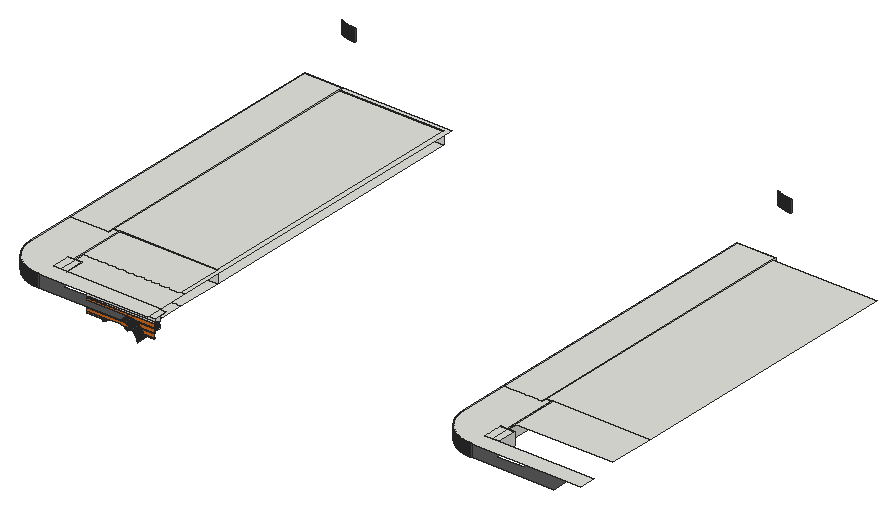
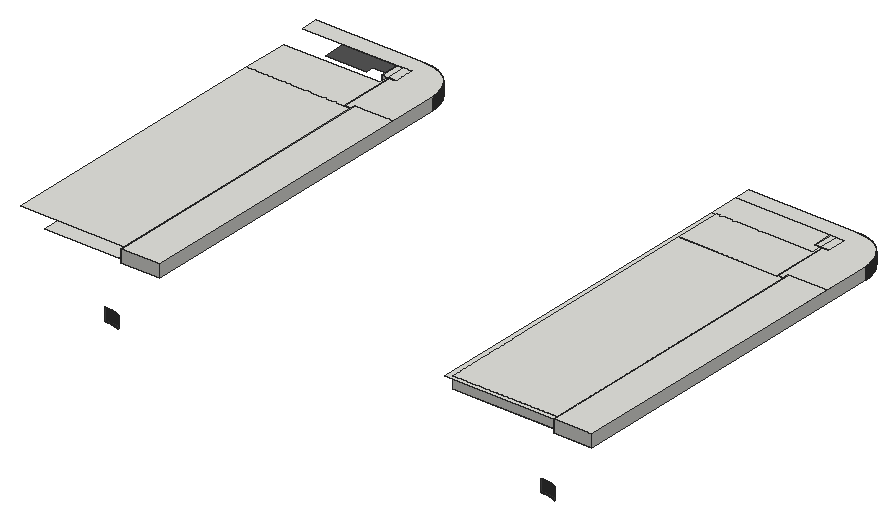
# SketchUp Ruby script. Lengths in inches.
U = 1.inch
M = Sketchup.active_model
def pt(a) = Geom::Point3d.new(a.map { |v| v * U })
def face(e, loops, mat)
  f = e.add_face(loops[0].map { |a| pt(a) })
  loops[1..].each { |l| e.add_face(l.map { |a| pt(a) }).erase! }
  f.material = f.back_material = mat if mat
  f
end
# faces: each face lists its corners as indices into pts; further lists are holes
def faces(e, pts, list, mat = nil) = list.each { |f| face(e, (f[0].is_a?(Array) ? f : [f]).map { |l| l.map { |i| pts[i] } }, mat) }
# xy, xz, yz: faces in a plane at the given z, y or x. An outline is a flat list of corners, or four numbers for a rectangle; further outlines are holes
def ring(l) = l.size == 4 ? [[l[0], l[1]], [l[2], l[1]], [l[2], l[3]], [l[0], l[3]]] : l.each_slice(2).to_a
def flat(e, list, mat, &to3) = list.each { |f| face(e, (f[0].is_a?(Array) ? f : [f]).map { |l| ring(l).map { |u, v| to3.(u, v) } }, mat) }
def xy(e, z, list, mat = nil) = flat(e, list, mat) { |x, y| [x, y, z] }
def xz(e, y, list, mat = nil) = flat(e, list, mat) { |x, z| [x, y, z] }
def yz(e, x, list, mat = nil) = flat(e, list, mat) { |y, z| [x, y, z] }
def lines(e, pts, list) = list.each { |a, b| e.add_line(pt(pts[a]), pt(pts[b])) }
# prism: a flat outline (further loops are holes) pulled along v
def prism(e, loops, v, mat = nil)
  f = face(e, loops, mat); d = Geom::Vector3d.new(v.map { |x| x * U })
  f.pushpull(f.normal.samedirection?(d) ? d.length : -d.length)
end
def box(e, o, s, mat = nil) = prism(e, [[o, [o[0] + s[0], o[1], o[2]], [o[0] + s[0], o[1] + s[1], o[2]], [o[0], o[1] + s[1], o[2]]]], [0, 0, s[2]], mat)
def at(x, y, z, deg = 0) = Geom::Transformation.translation(pt([x, y, z])) * Geom::Transformation.rotation(ORIGIN, Z_AXIS, deg.degrees)
def axes(o, x, y, z) = Geom::Transformation.new([*x, 0, *y, 0, *z, 0, *pt(o).to_a, 1])
def part(name) = M.definitions.add(name)
# library, detail: a bought-in or finely detailed component or shape, given as its bounding box
def library(name, o, s) = part(name).tap { |d| box(d.entities, o, s) }
def detail(e, o, s) = box(e.add_group.entities, o, s)
def put(e, d, t, mat = nil) = e.add_instance(d, t).tap { |i| i.material = mat if mat }
def group(e, t, mat = nil) = e.add_group.tap { |g| g.transformation = t; g.material = mat if mat }.entities
root = M.entities
M.materials.add("[0041_Chocolate]").color = [210, 105, 30]
M.materials.add("[Color M06]").color = [84, 84, 84]
xy(root,385.02,[[897.21,280.47,926.7,281.47],[954.52,280.47,998.64,281.47]],"[0041_Chocolate]")
xy(root,386.9375,[[897.21,280.47,931.67,281.47],[949.56,280.47,998.64,281.47]],"[0041_Chocolate]")
xy(root,391.89,[[897.21,280.47,998.64,281.47]],"[0041_Chocolate]")
xy(root,393.8125,[[897.21,280.47,998.64,281.47]],"[0041_Chocolate]")
xy(root,395.26,[[897.21,302.46,976.46,310.27]])
xy(root,398.77,[[897.21,280.47,998.64,281.47]],"[0041_Chocolate]")
xy(root,400.6875,[[897.21,280.47,998.64,281.47]],"[0041_Chocolate]")
xy(root,402.64,[[897.21,300.33,958.42,302.46],[990.02,302.46,992.73,302.46,992.73,337.5625,845.71,337.5625,845.71,321.34,857.24,321.34,857.24,305.58,897.21,305.58,897.21,312.8125,990.02,312.8125],[897.21,302.46,990.02,312.8125],[836,305.58,845.71,312.8125],[845.71,305.58,857.24,312.8125],
  [1486.5,305.58,1496.21,312.8125],[1496.21,305.58,1507.74,312.8125],[836,312.8125,845.71,321.34],[845.71,312.8125,857.24,321.34],[1486.5,312.8125,1496.21,321.34],
  [1496.21,312.8125,1507.74,321.34],[845.71,337.5625,992.73,406.38],[844.53,399.07,845.71,406.38],[1495.03,399.07,1496.21,406.38],[836,406.38,844.53,830.91],
  [844.53,406.38,955.73,830.91],[955.73,406.38,992.73,830.91],[1486.5,406.38,1495.03,830.91],[1495.03,406.38,1606.23,830.91]])
xy(root,402.64,[[834.95,267.75,833.46,267.77,831.97,267.83,830.49,267.93,829.01,268.0625,827.53,268.24,826.05,268.45,824.59,268.7,823.125,268.99,821.67,269.32,820.23,269.6875,818.8,270.09,817.375,270.53,815.96,271.01,814.57,271.53,813.18,272.08,811.8125,272.67,810.46,273.29,809.125,273.95,807.81,274.64,806.51,275.37,805.23,276.13,803.97,276.93,802.73,277.75,801.51,278.61,800.32,279.51,799.15,280.43,798.01,281.38,796.89,282.36,795.79,283.37,794.73,284.41,793.6875,285.48,792.68,286.57,791.69,287.69,790.74,288.84,789.82,290.01,788.93,291.2,788.07,292.42,787.24,293.65,786.45,294.91,785.6875,296.19,784.96,297.49,784.27,298.8125,783.61,300.15,782.98,301.5,782.4,302.87,781.84,304.25,781.33,305.65,780.85,307.06,780.41,308.48,780,309.91,779.64,311.36,779.31,312.81,779.02,314.27,778.77,315.74,778.55,317.21,778.375,318.69,778.24,320.17,778.14,321.66,778.08,323.15,778.07,324.64,778.07,838.14,836,838.14,836,305.58,857.24,305.58,857.24,287.95,897.21,287.95,897.21,300.33,958.42,300.33,958.42,267.75],[1485.45,267.75,1483.96,267.77,1482.47,267.83,1480.99,267.93,1479.51,268.0625,1478.03,268.24,1476.55,268.45,1475.09,268.7,1473.625,268.99,1472.17,269.32,1470.73,269.6875,1469.3,270.09,1467.875,270.53,1466.46,271.01,1465.07,271.53,1463.68,272.08,1462.3125,272.67,1460.96,273.29,1459.625,273.95,1458.31,274.64,1457.01,275.37,1455.73,276.13,1454.47,276.93,1453.23,277.75,1452.01,278.61,1450.82,279.51,1449.65,280.43,1448.51,281.38,1447.39,282.36,1446.29,283.37,1445.23,284.41,1444.1875,285.48,1443.18,286.57,1442.19,287.69,1441.24,288.84,1440.32,290.01,1439.43,291.2,1438.57,292.42,1437.74,293.65,1436.95,294.91,1436.1875,296.19,1435.46,297.49,1434.77,298.8125,1434.11,300.15,1433.48,301.5,1432.9,302.87,1432.34,304.25,1431.83,305.65,1431.35,307.06,1430.91,308.48,1430.5,309.91,1430.14,311.36,1429.81,312.81,1429.52,314.27,1429.27,315.74,1429.05,317.21,1428.875,318.69,1428.74,320.17,1428.64,321.66,1428.58,323.15,1428.57,324.64,1428.57,838.14,1486.5,838.14,1486.5,305.58,1507.74,305.58,1507.74,287.95,1547.71,287.95,1547.71,300.33,1608.92,300.33,1608.92,267.75]],"[Color M06]")
xy(root,405.64,[[897.21,280.47,998.64,281.47]],"[0041_Chocolate]")
xy(root,411.82,[[897.21,281.47,998.64,302.46]])
xy(root,421.25,[[834.95,267.75,999.52,267.75,999.52,292.45,836,292.45,836,321.34,844.53,321.34,844.53,406.38,836,406.38,836,397.86,778.07,397.86,778.07,324.64,778.08,323.15,778.14,321.66,778.24,320.17,778.375,318.69,778.55,317.21,778.77,315.74,779.02,314.27,779.31,312.81,779.64,311.36,780,309.91,780.41,308.48,780.85,307.06,781.33,305.65,781.84,304.25,782.4,302.87,782.98,301.5,783.61,300.15,784.27,298.8125,784.96,297.49,785.6875,296.19,786.45,294.91,787.24,293.65,788.07,292.42,788.93,291.2,789.82,290.01,790.74,288.84,791.69,287.69,792.68,286.57,793.6875,285.48,794.73,284.41,795.79,283.37,796.89,282.36,798.01,281.38,799.15,280.43,800.32,279.51,801.51,278.61,802.73,277.75,803.97,276.93,805.23,276.13,806.51,275.37,807.81,274.64,809.125,273.95,810.46,273.29,811.8125,272.67,813.18,272.08,814.57,271.53,815.96,271.01,817.375,270.53,818.8,270.09,820.23,269.6875,821.67,269.32,823.125,268.99,824.59,268.7,826.05,268.45,827.53,268.24,829.01,268.0625,830.49,267.93,831.97,267.83,833.46,267.77],[1485.45,267.75,1650.02,267.75,1650.02,292.45,1486.5,292.45,1486.5,321.34,1495.03,321.34,1495.03,406.38,1486.5,406.38,1486.5,397.86,1428.57,397.86,1428.57,324.64,1428.58,323.15,1428.64,321.66,1428.74,320.17,1428.875,318.69,1429.05,317.21,1429.27,315.74,1429.52,314.27,1429.81,312.81,1430.14,311.36,1430.5,309.91,1430.91,308.48,1431.35,307.06,1431.83,305.65,1432.34,304.25,1432.9,302.87,1433.48,301.5,1434.11,300.15,1434.77,298.8125,1435.46,297.49,1436.1875,296.19,1436.95,294.91,1437.74,293.65,1438.57,292.42,1439.43,291.2,1440.32,290.01,1441.24,288.84,1442.19,287.69,1443.18,286.57,1444.1875,285.48,1445.23,284.41,1446.29,283.37,1447.39,282.36,1448.51,281.38,1449.65,280.43,1450.82,279.51,1452.01,278.61,1453.23,277.75,1454.47,276.93,1455.73,276.13,1457.01,275.37,1458.31,274.64,1459.625,273.95,1460.96,273.29,1462.3125,272.67,1463.68,272.08,1465.07,271.53,1466.46,271.01,1467.875,270.53,1469.3,270.09,1470.73,269.6875,1472.17,269.32,1473.625,268.99,1475.09,268.7,1476.55,268.45,1478.03,268.24,1479.51,268.0625,1480.99,267.93,1482.47,267.83,1483.96,267.77],[836,292.45,847.59,321.34],[847.59,292.45,857.24,321.34],[857.24,292.45,999.52,292.45,999.52,336.27,847.59,336.27,847.59,321.34,857.24,321.34],
  [1486.5,292.45,1498.09,321.34],[1498.09,292.45,1507.74,321.34],[844.53,321.34,845.71,406.38],[845.71,321.34,847.59,321.34,847.59,336.27,992.73,336.27,992.73,406.38,845.71,406.38],[1495.03,321.34,1496.21,406.38],
  [1496.21,321.34,1498.09,321.34,1498.09,336.27,1643.23,336.27,1643.23,406.38,1496.21,406.38],[992.73,336.27,999.52,336.27,999.52,838.14,836,838.14,836,830.91,992.73,830.91],[778.07,397.86,836,838.14],[1428.57,397.86,1486.5,838.14],[836,406.38,992.73,830.91],
  [1486.5,406.38,1643.23,830.91]])
xz(root,280.47,[[897.21,386.9375,931.67,386.9375,936.5,388.23,944.69,388.24,949.56,386.9375,998.64,386.9375,998.64,391.89,897.21,391.89],[897.21,393.8125,998.64,398.77],[897.21,400.6875,998.64,405.64]],"[0041_Chocolate]")
xz(root,281.47,[[897.21,405.64,998.64,407.5625],[897.21,407.5625,998.64,411.82],[897.21,411.82,998.64,412.52]])
xz(root,281.47,[[897.21,385.02,926.7,385.02,928.6,386.11,931.67,386.9375,897.21,386.9375],[954.52,385.02,998.64,385.02,998.64,386.9375,949.56,386.9375,952.6,386.125],[897.21,391.89,998.64,393.8125],[897.21,398.77,998.64,400.6875]],"[0041_Chocolate]")
xz(root,302.46,[[897.21,395.26,976.46,395.26,976.15,395.5625,975.66,396.02,975.15,396.46,974.63,396.89,974.1,397.3125,973.56,397.72,973.01,398.1,972.45,398.48,971.88,398.84,971.3,399.18,970.71,399.51,970.11,399.83,969.51,400.125,968.9,400.41,968.28,400.67,967.65,400.92,967.02,401.16,966.38,401.375,965.74,401.57,965.09,401.76,964.43,401.92,963.77,402.07,963.11,402.2,962.45,402.32,961.78,402.41,961.11,402.49,960.44,402.56,959.77,402.6,959.09,402.625,958.42,402.64,897.21,402.64],[976.46,395.26,984.18,395.26,984.18,402.64,958.42,402.64,959.09,402.625,959.77,402.6,960.44,402.56,961.11,402.49,961.78,402.41,962.45,402.32,963.11,402.2,963.77,402.07,964.43,401.92,965.09,401.76,965.74,401.57,966.38,401.375,967.02,401.16,967.65,400.92,968.28,400.67,968.9,400.41,969.51,400.125,970.11,399.83,970.71,399.51,971.3,399.18,971.88,398.84,972.45,398.48,973.01,398.1,973.56,397.72,974.1,397.3125,974.63,396.89,975.15,396.46,975.66,396.02,976.15,395.5625],[984.18,395.26,990.02,402.64],[897.21,402.64,984.18,411.82]])
xz(root,321.34,[[836,402.64,844.53,421.25],[844.53,402.64,845.71,421.25],[845.71,402.64,847.59,421.25],[847.59,402.64,857.24,421.25],[1486.5,402.64,1495.03,421.25],
  [1495.03,402.64,1496.21,421.25],[1496.21,402.64,1498.09,421.25],[1498.09,402.64,1507.74,421.25]])
xz(root,406.38,[[836,402.64,844.53,421.25],[844.53,402.64,845.71,421.25],[845.71,402.64,992.73,421.25],[1486.5,402.64,1495.03,421.25],[1495.03,402.64,1496.21,421.25]])
xz(root,830.91,[[836,402.64,992.73,421.25]])
xz(root,838.14,[[778.07,402.64,836,421.25],[1428.57,402.64,1486.5,421.25]])
yz(root,778.07,[[324.64,402.64,838.14,421.25]])
yz(root,836,[[397.86,402.64,406.38,421.25],[406.38,402.64,830.91,421.25],[830.91,402.64,838.14,421.25]])
yz(root,845.71,[[321.34,402.64,406.38,421.25]])
yz(root,857.24,[[292.45,402.64,321.34,421.25]])
yz(root,897.21,[[300.33,395.26,302.46,402.64],[302.46,395.26,305.58,402.64]])
yz(root,1428.57,[[324.64,402.64,838.14,421.25]])
yz(root,1486.5,[[397.86,402.64,406.38,421.25],[406.38,402.64,830.91,421.25],[830.91,402.64,838.14,421.25]])
yz(root,1496.21,[[321.34,402.64,406.38,421.25]])
yz(root,1507.74,[[292.45,402.64,321.34,421.25]])
p = [[983.75,267.75,381.57],[983.75,302.46,381.57],[983.86,302.46,380.9],[983.86,267.75,380.9],[983.86,310.27,380.9],[983.75,310.27,381.57],
  [983.62,267.75,382.23],[983.62,302.46,382.23],[983.62,310.27,382.23],[926.7,295.65,385.02],[926.7,281.47,385.02],[926.7,280.47,385.02],
  [921.51,280.47,382.01],[921.51,295.65,382.01],[959.69,295.65,382.03],[959.69,280.47,382.03],[954.52,280.47,385.02],[954.52,281.47,385.02],
  [954.52,295.65,385.02],[983.47,267.75,382.89],[983.47,302.46,382.89],[983.47,310.27,382.89],[983.3,267.75,383.54],[983.3,302.46,383.54],
  [983.3,310.27,383.54],[983.12,267.75,384.19],[983.12,302.46,384.19],[983.28,302.46,383.64],[983.28,310.27,383.64],[983.12,310.27,384.19],
  [982.92,267.75,384.84],[982.92,302.46,384.84],[982.92,310.27,384.84],[982.7,267.75,385.47],[982.7,302.46,385.47],[982.7,310.27,385.47],
  [928.6,281.47,386.11],[928.6,295.65,386.11],[952.6,281.47,386.125],[952.6,295.65,386.125],[982.47,267.75,386.11],[982.47,302.46,386.11],
  [982.6,302.46,385.76],[982.6,310.27,385.76],[982.47,310.27,386.11],[982.22,267.75,386.73],[982.22,302.46,386.73],[931.67,281.47,386.9375],
  [931.67,295.65,386.9375],[949.56,281.47,386.9375],[949.56,295.65,386.9375],[982.22,310.27,386.73],[981.95,267.75,387.35],[981.95,302.46,387.35],
  [981.95,310.27,387.35],[936.5,295.65,388.23],[936.5,280.47,388.23],[931.67,280.47,386.9375],[949.56,280.47,386.9375],[944.69,280.47,388.24],
  [944.69,295.65,388.24],[981.67,267.75,387.96],[981.67,302.46,387.96],[981.67,310.27,387.96],[981.37,267.75,388.57],[981.37,302.46,388.57],
  [981.37,310.27,388.57],[981.06,267.75,389.17],[981.06,302.46,389.17],[981.06,310.27,389.17],[980.73,267.75,389.76],[980.73,302.46,389.76],
  [980.73,310.27,389.76],[980.38,267.75,390.33],[980.38,302.46,390.33],[980.38,310.27,390.33],[980.02,267.75,390.9],[980.02,302.46,390.9],
  [980.02,310.27,390.9],[979.65,267.75,391.47],[979.65,302.46,391.47],[979.65,310.27,391.47],[979.26,267.75,392.02],[979.26,302.46,392.02],
  [979.26,310.27,392.02],[978.86,267.75,392.56],[978.86,302.46,392.56],[978.86,310.27,392.56],[978.4375,267.75,393.09],[978.4375,302.46,393.09],
  [978.4375,310.27,393.09],[978.01,267.75,393.6],[978.01,302.46,393.6],[978.4,302.46,393.14],[978.4,310.27,393.14],[978.01,310.27,393.6],
  [977.5625,267.75,394.11],[977.5625,302.46,394.11],[977.5625,310.27,394.11],[977.1,267.75,394.61],[977.1,302.46,394.61],[977.1,310.27,394.61],
  [976.63,267.75,395.09],[976.63,302.46,395.09],[976.63,310.27,395.09],[976.15,267.75,395.5625],[976.15,300.33,395.5625],[976.46,300.33,395.26],
  [976.46,302.46,395.26],[976.46,310.27,395.26],[976.15,302.46,395.5625],[975.66,267.75,396.02],[975.66,300.33,396.02],[975.66,302.46,396.02],
  [975.15,267.75,396.46],[975.15,300.33,396.46],[975.15,302.46,396.46],[974.63,267.75,396.89],[974.63,300.33,396.89],[974.63,302.46,396.89],
  [974.1,267.75,397.3125],[974.1,300.33,397.3125],[974.1,302.46,397.3125],[973.56,267.75,397.72],[973.56,300.33,397.72],[973.56,302.46,397.72],
  [973.01,267.75,398.1],[973.01,300.33,398.1],[973.01,302.46,398.1],[972.45,267.75,398.48],[972.45,300.33,398.48],[972.45,302.46,398.48],
  [971.88,267.75,398.84],[971.88,300.33,398.84],[971.88,302.46,398.84],[971.3,267.75,399.18],[971.3,300.33,399.18],[971.3,302.46,399.18],
  [970.71,267.75,399.51],[970.71,300.33,399.51],[970.71,302.46,399.51],[970.11,267.75,399.83],[970.11,300.33,399.83],[970.11,302.46,399.83],
  [969.51,267.75,400.125],[969.51,300.33,400.125],[969.51,302.46,400.125],[968.9,267.75,400.41],[968.9,300.33,400.41],[968.9,302.46,400.41],
  [968.28,267.75,400.67],[968.28,300.33,400.67],[968.28,302.46,400.67],[967.65,267.75,400.92],[967.65,300.33,400.92],[967.65,302.46,400.92],
  [967.02,267.75,401.16],[967.02,300.33,401.16],[967.02,302.46,401.16],[966.38,267.75,401.375],[966.38,300.33,401.375],[966.38,302.46,401.375],
  [965.74,267.75,401.57],[965.74,300.33,401.57],[965.74,302.46,401.57],[965.09,267.75,401.76],[965.09,300.33,401.76],[965.09,302.46,401.76],
  [964.43,267.75,401.92],[964.43,300.33,401.92],[964.43,302.46,401.92],[963.77,267.75,402.07],[963.77,300.33,402.07],[963.77,302.46,402.07],
  [963.11,267.75,402.2],[963.11,300.33,402.2],[963.11,302.46,402.2],[962.45,267.75,402.32],[962.45,300.33,402.32],[962.45,302.46,402.32],
  [961.78,267.75,402.41],[961.78,300.33,402.41],[961.78,302.46,402.41],[961.11,267.75,402.49],[961.11,300.33,402.49],[961.11,302.46,402.49],
  [960.44,267.75,402.56],[960.44,300.33,402.56],[960.44,302.46,402.56],[831.97,267.83,421.25],[830.49,267.93,421.25],[830.49,267.93,402.64],
  [831.97,267.83,402.64],[833.46,267.77,421.25],[833.46,267.77,402.64],[834.95,267.75,421.25],[834.95,267.75,402.64],[958.42,267.75,402.64],
  [958.42,300.33,402.64],[959.09,300.33,402.625],[959.09,267.75,402.625],[959.77,300.33,402.6],[959.77,267.75,402.6],[1482.47,267.83,421.25],
  [1480.99,267.93,421.25],[1480.99,267.93,402.64],[1482.47,267.83,402.64],[1483.96,267.77,421.25],[1483.96,267.77,402.64],[1485.45,267.75,421.25],
  [1485.45,267.75,402.64],[829.01,268.0625,421.25],[829.01,268.0625,402.64],[1479.51,268.0625,421.25],[1479.51,268.0625,402.64],[827.53,268.24,421.25],
  [827.53,268.24,402.64],[1478.03,268.24,421.25],[1478.03,268.24,402.64],[826.05,268.45,421.25],[826.05,268.45,402.64],[1476.55,268.45,421.25],
  [1476.55,268.45,402.64],[824.59,268.7,421.25],[824.59,268.7,402.64],[1475.09,268.7,421.25],[1475.09,268.7,402.64],[823.125,268.99,421.25],
  [823.125,268.99,402.64],[1473.625,268.99,421.25],[1473.625,268.99,402.64],[821.67,269.32,421.25],[821.67,269.32,402.64],[1472.17,269.32,421.25],
  [1472.17,269.32,402.64],[820.23,269.6875,421.25],[820.23,269.6875,402.64],[1470.73,269.6875,421.25],[1470.73,269.6875,402.64],[818.8,270.09,421.25],
  [818.8,270.09,402.64],[1469.3,270.09,421.25],[1469.3,270.09,402.64],[817.375,270.53,421.25],[817.375,270.53,402.64],[1467.875,270.53,421.25],
  [1467.875,270.53,402.64],[815.96,271.01,421.25],[815.96,271.01,402.64],[1466.46,271.01,421.25],[1466.46,271.01,402.64],[814.57,271.53,421.25],
  [814.57,271.53,402.64],[1465.07,271.53,421.25],[1465.07,271.53,402.64],[813.18,272.08,421.25],[813.18,272.08,402.64],[1463.68,272.08,421.25],
  [1463.68,272.08,402.64],[811.8125,272.67,421.25],[811.8125,272.67,402.64],[1462.3125,272.67,421.25],[1462.3125,272.67,402.64],[810.46,273.29,421.25],
  [810.46,273.29,402.64],[1460.96,273.29,421.25],[1460.96,273.29,402.64],[809.125,273.95,421.25],[809.125,273.95,402.64],[1459.625,273.95,421.25],
  [1459.625,273.95,402.64],[807.81,274.64,421.25],[807.81,274.64,402.64],[1458.31,274.64,421.25],[1458.31,274.64,402.64],[806.51,275.37,421.25],
  [806.51,275.37,402.64],[1457.01,275.37,421.25],[1457.01,275.37,402.64],[805.23,276.13,421.25],[805.23,276.13,402.64],[1455.73,276.13,421.25],
  [1455.73,276.13,402.64],[803.97,276.93,421.25],[803.97,276.93,402.64],[1454.47,276.93,421.25],[1454.47,276.93,402.64],[802.73,277.75,421.25],
  [802.73,277.75,402.64],[1453.23,277.75,421.25],[1453.23,277.75,402.64],[801.51,278.61,421.25],[801.51,278.61,402.64],[1452.01,278.61,421.25],
  [1452.01,278.61,402.64],[800.32,279.51,421.25],[800.32,279.51,402.64],[1450.82,279.51,421.25],[1450.82,279.51,402.64],[799.15,280.43,421.25],
  [799.15,280.43,402.64],[1449.65,280.43,421.25],[1449.65,280.43,402.64],[798.01,281.38,421.25],[798.01,281.38,402.64],[1448.51,281.38,421.25],
  [1448.51,281.38,402.64],[796.89,282.36,421.25],[796.89,282.36,402.64],[1447.39,282.36,421.25],[1447.39,282.36,402.64],[795.79,283.37,421.25],
  [795.79,283.37,402.64],[1446.29,283.37,421.25],[1446.29,283.37,402.64],[794.73,284.41,421.25],[794.73,284.41,402.64],[1445.23,284.41,421.25],
  [1445.23,284.41,402.64],[793.6875,285.48,421.25],[793.6875,285.48,402.64],[1444.1875,285.48,421.25],[1444.1875,285.48,402.64],[792.68,286.57,421.25],
  [792.68,286.57,402.64],[1443.18,286.57,421.25],[1443.18,286.57,402.64],[791.69,287.69,421.25],[791.69,287.69,402.64],[1442.19,287.69,421.25],
  [1442.19,287.69,402.64],[790.74,288.84,421.25],[790.74,288.84,402.64],[1441.24,288.84,421.25],[1441.24,288.84,402.64],[789.82,290.01,421.25],
  [789.82,290.01,402.64],[1440.32,290.01,421.25],[1440.32,290.01,402.64],[788.93,291.2,421.25],[788.93,291.2,402.64],[1439.43,291.2,421.25],
  [1439.43,291.2,402.64],[788.07,292.42,421.25],[788.07,292.42,402.64],[1438.57,292.42,421.25],[1438.57,292.42,402.64],[787.24,293.65,421.25],
  [787.24,293.65,402.64],[1437.74,293.65,421.25],[1437.74,293.65,402.64],[786.45,294.91,421.25],[786.45,294.91,402.64],[1436.95,294.91,421.25],
  [1436.95,294.91,402.64],[785.6875,296.19,421.25],[785.6875,296.19,402.64],[1436.1875,296.19,421.25],[1436.1875,296.19,402.64],[784.96,297.49,421.25],
  [784.96,297.49,402.64],[1435.46,297.49,421.25],[1435.46,297.49,402.64],[784.27,298.8125,421.25],[784.27,298.8125,402.64],[1434.77,298.8125,421.25],
  [1434.77,298.8125,402.64],[783.61,300.15,421.25],[783.61,300.15,402.64],[1434.11,300.15,421.25],[1434.11,300.15,402.64],[782.98,301.5,421.25],
  [782.98,301.5,402.64],[1433.48,301.5,421.25],[1433.48,301.5,402.64],[958.42,302.46,402.64],[959.09,302.46,402.625],[959.77,302.46,402.6],
  [782.4,302.87,421.25],[782.4,302.87,402.64],[1432.9,302.87,421.25],[1432.9,302.87,402.64],[781.84,304.25,421.25],[781.84,304.25,402.64],
  [1432.34,304.25,421.25],[1432.34,304.25,402.64],[781.33,305.65,421.25],[781.33,305.65,402.64],[1431.83,305.65,421.25],[1431.83,305.65,402.64],
  [780.85,307.06,421.25],[780.85,307.06,402.64],[1431.35,307.06,421.25],[1431.35,307.06,402.64],[780.41,308.48,421.25],[780.41,308.48,402.64],
  [1430.91,308.48,421.25],[1430.91,308.48,402.64],[780,309.91,421.25],[780,309.91,402.64],[1430.5,309.91,421.25],[1430.5,309.91,402.64],
  [779.64,311.36,421.25],[779.64,311.36,402.64],[1430.14,311.36,421.25],[1430.14,311.36,402.64],[779.31,312.81,421.25],[779.31,312.81,402.64],
  [1429.81,312.81,421.25],[1429.81,312.81,402.64],[779.02,314.27,421.25],[779.02,314.27,402.64],[1429.52,314.27,421.25],[1429.52,314.27,402.64],
  [778.77,315.74,421.25],[778.77,315.74,402.64],[1429.27,315.74,421.25],[1429.27,315.74,402.64],[778.55,317.21,421.25],[778.55,317.21,402.64],
  [1429.05,317.21,421.25],[1429.05,317.21,402.64],[778.375,318.69,421.25],[778.375,318.69,402.64],[1428.875,318.69,421.25],[1428.875,318.69,402.64],
  [778.24,320.17,421.25],[778.24,320.17,402.64],[1428.74,320.17,421.25],[1428.74,320.17,402.64],[778.14,321.66,421.25],[778.14,321.66,402.64],
  [1428.64,321.66,421.25],[1428.64,321.66,402.64],[778.08,323.15,421.25],[778.08,323.15,402.64],[1428.58,323.15,421.25],[1428.58,323.15,402.64],
  [778.07,324.64,421.25],[778.07,324.64,402.64],[1428.57,324.64,421.25],[1428.57,324.64,402.64],[758.26,958.64,421.25],[756.78,958.66,421.25],
  [756.78,958.66,402.64],[758.26,958.64,402.64],[1413.76,958.64,421.25],[1412.28,958.66,421.25],[1412.28,958.66,402.64],[1413.76,958.64,402.64],
  [755.29,958.72,421.25],[753.8,958.82,421.25],[753.8,958.82,402.64],[755.29,958.72,402.64],[1410.79,958.72,421.25],[1409.3,958.82,421.25],
  [1409.3,958.82,402.64],[1410.79,958.72,402.64],[752.32,958.96,421.25],[752.32,958.96,402.64],[1407.82,958.96,421.25],[1407.82,958.96,402.64],
  [750.84,959.13,421.25],[750.84,959.13,402.64],[1406.34,959.13,421.25],[1406.34,959.13,402.64],[749.37,959.34,421.25],[749.37,959.34,402.64],
  [1404.87,959.34,421.25],[1404.87,959.34,402.64],[747.9,959.6,421.25],[747.9,959.6,402.64],[1403.4,959.6,421.25],[1403.4,959.6,402.64],
  [746.4375,959.89,421.25],[746.4375,959.89,402.64],[1401.9375,959.89,421.25],[1401.9375,959.89,402.64],[744.98,960.22,421.25],[744.98,960.22,402.64],
  [1400.48,960.22,421.25],[1400.48,960.22,402.64],[743.54,960.58,421.25],[743.54,960.58,402.64],[1399.04,960.58,421.25],[1399.04,960.58,402.64],
  [742.11,960.99,421.25],[742.11,960.99,402.64],[1397.61,960.99,421.25],[1397.61,960.99,402.64],[740.6875,961.43,421.25],[740.6875,961.43,402.64],
  [1396.1875,961.43,421.25],[1396.1875,961.43,402.64],[739.28,961.91,421.25],[739.28,961.91,402.64],[1394.78,961.91,421.25],[1394.78,961.91,402.64],
  [737.88,962.42,421.25],[737.88,962.42,402.64],[1393.38,962.42,421.25],[1393.38,962.42,402.64],[736.49,962.97,421.25],[736.49,962.97,402.64],
  [1391.99,962.97,421.25],[1391.99,962.97,402.64],[735.125,963.5625,421.25],[735.125,963.5625,402.64],[1390.625,963.5625,421.25],[1390.625,963.5625,402.64],
  [733.77,964.1875,421.25],[733.77,964.1875,402.64],[1389.27,964.1875,421.25],[1389.27,964.1875,402.64]]
faces(root,p,[[0,1,2,3],[6,7,1,0],[19,20,7,6],[22,23,20,19],[25,26,27,23,22],[30,31,26,25],[33,34,31,30],[40,41,42,34,33],
  [45,46,41,40],[52,53,46,45],[61,62,53,52],[64,65,62,61],[67,68,65,64],[70,71,68,67],[73,74,71,70],[76,77,74,73],
  [79,80,77,76],[82,83,80,79],[85,86,83,82],[88,89,86,85],[91,92,93,89,88],[96,97,92,91],[99,100,97,96],[102,103,100,99],
  [105,106,107,108,103,102],[111,112,106,105],[114,115,112,111],[117,118,115,114],[120,121,118,117],[123,124,121,120],[126,127,124,123],[129,130,127,126],
  [132,133,130,129],[135,136,133,132],[138,139,136,135],[141,142,139,138],[144,145,142,141],[147,148,145,144],[150,151,148,147],[153,154,151,150],
  [156,157,154,153],[159,160,157,156],[162,163,160,159],[165,166,163,162],[168,169,166,165],[171,172,169,168],[174,175,172,171],[177,178,175,174],
  [180,181,178,177],[183,184,181,180],[186,187,184,183],[189,190,191,192],[193,189,192,194],[195,193,194,196],[197,198,199,200],[200,199,201,202],
  [202,201,187,186],[203,204,205,206],[207,203,206,208],[209,207,208,210],[190,211,212,191],[204,213,214,205],[211,215,216,212],[213,217,218,214],
  [215,219,220,216],[217,221,222,218],[219,223,224,220],[221,225,226,222],[223,227,228,224],[225,229,230,226],[227,231,232,228],[229,233,234,230],
  [231,235,236,232],[233,237,238,234],[235,239,240,236],[237,241,242,238],[239,243,244,240],[241,245,246,242],[243,247,248,244],[245,249,250,246],
  [247,251,252,248],[249,253,254,250],[251,255,256,252],[253,257,258,254],[255,259,260,256],[257,261,262,258],[259,263,264,260],[261,265,266,262],
  [263,267,268,264],[265,269,270,266],[267,271,272,268],[269,273,274,270],[271,275,276,272],[273,277,278,274],[275,279,280,276],[277,281,282,278],
  [279,283,284,280],[281,285,286,282],[283,287,288,284],[285,289,290,286],[287,291,292,288],[289,293,294,290],[291,295,296,292],[293,297,298,294],
  [295,299,300,296],[297,301,302,298],[299,303,304,300],[301,305,306,302],[303,307,308,304],[305,309,310,306],[307,311,312,308],[309,313,314,310],
  [311,315,316,312],[313,317,318,314],[315,319,320,316],[317,321,322,318],[319,323,324,320],[321,325,326,322],[323,327,328,324],[325,329,330,326],
  [327,331,332,328],[329,333,334,330],[331,335,336,332],[333,337,338,334],[335,339,340,336],[337,341,342,338],[339,343,344,340],[341,345,346,342],
  [343,347,348,344],[345,349,350,346],[347,351,352,348],[349,353,354,350],[351,355,356,352],[353,357,358,354],[355,359,360,356],[357,361,362,358],
  [359,363,364,360],[361,365,366,362],[363,367,368,364],[365,369,370,366],[367,371,372,368],[369,373,374,370],[371,378,379,372],[373,380,381,374],
  [378,382,383,379],[380,384,385,381],[382,386,387,383],[384,388,389,385],[386,390,391,387],[388,392,393,389],[390,394,395,391],[392,396,397,393],
  [394,398,399,395],[396,400,401,397],[398,402,403,399],[400,404,405,401],[402,406,407,403],[404,408,409,405],[406,410,411,407],[408,412,413,409],
  [410,414,415,411],[412,416,417,413],[414,418,419,415],[416,420,421,417],[418,422,423,419],[420,424,425,421],[422,426,427,423],[424,428,429,425],
  [426,430,431,427],[428,432,433,429],[430,434,435,431],[432,436,437,433],[434,438,439,435],[436,440,441,437],[442,443,444,445],[446,447,448,449],
  [450,451,452,453],[443,450,453,444],[454,455,456,457],[447,454,457,448],[451,458,459,452],[455,460,461,456],[458,462,463,459],[460,464,465,461],
  [462,466,467,463],[464,468,469,465],[466,470,471,467],[468,472,473,469],[470,474,475,471],[472,476,477,473],[474,478,479,475],[476,480,481,477],
  [478,482,483,479],[480,484,485,481],[482,486,487,483],[484,488,489,485],[486,490,491,487],[488,492,493,489],[490,494,495,491],[492,496,497,493],
  [494,498,499,495],[496,500,501,497],[498,502,503,499],[500,504,505,501],[502,506,507,503],[504,508,509,505],[506,510,511,507],[508,512,513,509]],"[Color M06]")
faces(root,p,[[1,2,4,5],[7,1,5,8],[9,10,11,12,13],[14,15,16,17,18],[20,7,8,21],[23,20,21,24],[27,23,24,28],[26,27,28,29],
  [31,26,29,32],[34,31,32,35],[36,10,9,37],[17,38,39,18],[42,34,35,43],[41,42,43,44],[47,36,37,48],[38,49,50,39],
  [46,41,44,51],[53,46,51,54],[55,56,57,47,48],[50,49,58,59,60],[62,53,54,63],[65,62,63,66],[60,59,56,55],[68,65,66,69],
  [71,68,69,72],[74,71,72,75],[77,74,75,78],[80,77,78,81],[83,80,81,84],[86,83,84,87],[89,86,87,90],[92,93,94,95],
  [93,89,90,94],[97,92,95,98],[100,97,98,101],[103,100,101,104],[108,103,104,109],[110,108,107,106],[113,110,106,112],[116,113,112,115],
  [119,116,115,118],[122,119,118,121],[125,122,121,124],[128,125,124,127],[131,128,127,130],[134,131,130,133],[137,134,133,136],[140,137,136,139],
  [143,140,139,142],[146,143,142,145],[149,146,145,148],[152,149,148,151],[155,152,151,154],[158,155,154,157],[161,158,157,160],[164,161,160,163],
  [167,164,163,166],[170,167,166,169],[173,170,169,172],[176,173,172,175],[179,176,175,178],[182,179,178,181],[185,182,181,184],[188,185,184,187],
  [375,376,199,198],[376,377,201,199],[377,188,187,201]])
